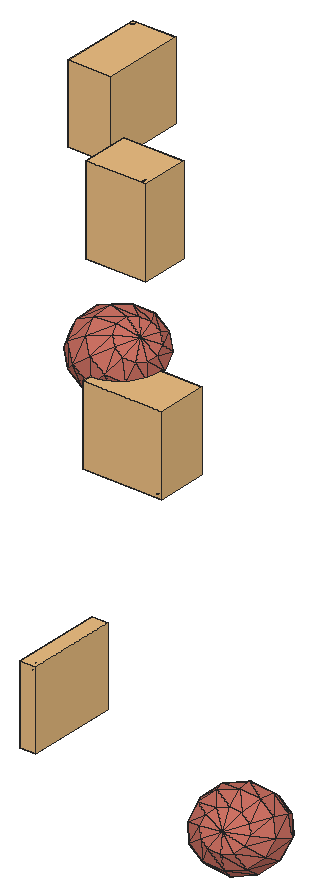
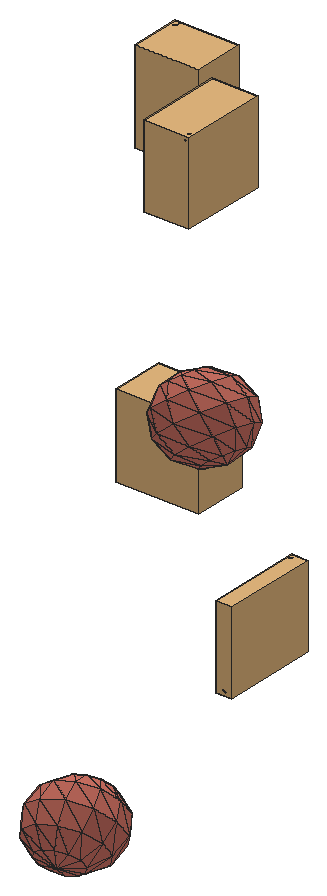
# SketchUp Ruby script. Lengths in inches.
U = 1.inch
M = Sketchup.active_model
def pt(a) = Geom::Point3d.new(a.map { |v| v * U })
def face(e, loops, mat)
  f = e.add_face(loops[0].map { |a| pt(a) })
  loops[1..].each { |l| e.add_face(l.map { |a| pt(a) }).erase! }
  f.material = f.back_material = mat if mat
  f
end
# faces: each face lists its corners as indices into pts; further lists are holes
def faces(e, pts, list, mat = nil) = list.each { |f| face(e, (f[0].is_a?(Array) ? f : [f]).map { |l| l.map { |i| pts[i] } }, mat) }
# xy, xz, yz: faces in a plane at the given z, y or x. An outline is a flat list of corners, or four numbers for a rectangle; further outlines are holes
def ring(l) = l.size == 4 ? [[l[0], l[1]], [l[2], l[1]], [l[2], l[3]], [l[0], l[3]]] : l.each_slice(2).to_a
def flat(e, list, mat, &to3) = list.each { |f| face(e, (f[0].is_a?(Array) ? f : [f]).map { |l| ring(l).map { |u, v| to3.(u, v) } }, mat) }
def xy(e, z, list, mat = nil) = flat(e, list, mat) { |x, y| [x, y, z] }
def xz(e, y, list, mat = nil) = flat(e, list, mat) { |x, z| [x, y, z] }
def yz(e, x, list, mat = nil) = flat(e, list, mat) { |y, z| [x, y, z] }
def lines(e, pts, list) = list.each { |a, b| e.add_line(pt(pts[a]), pt(pts[b])) }
# prism: a flat outline (further loops are holes) pulled along v
def prism(e, loops, v, mat = nil)
  f = face(e, loops, mat); d = Geom::Vector3d.new(v.map { |x| x * U })
  f.pushpull(f.normal.samedirection?(d) ? d.length : -d.length)
end
def box(e, o, s, mat = nil) = prism(e, [[o, [o[0] + s[0], o[1], o[2]], [o[0] + s[0], o[1] + s[1], o[2]], [o[0], o[1] + s[1], o[2]]]], [0, 0, s[2]], mat)
def at(x, y, z, deg = 0) = Geom::Transformation.translation(pt([x, y, z])) * Geom::Transformation.rotation(ORIGIN, Z_AXIS, deg.degrees)
def axes(o, x, y, z) = Geom::Transformation.new([*x, 0, *y, 0, *z, 0, *pt(o).to_a, 1])
def part(name) = M.definitions.add(name)
# library, detail: a bought-in or finely detailed component or shape, given as its bounding box
def library(name, o, s) = part(name).tap { |d| box(d.entities, o, s) }
def detail(e, o, s) = box(e.add_group.entities, o, s)
def put(e, d, t, mat = nil) = e.add_instance(d, t).tap { |i| i.material = mat if mat }
def group(e, t, mat = nil) = e.add_group.tap { |g| g.transformation = t; g.material = mat if mat }.entities
root = M.entities
M.materials.add("green").color = [174, 139, 102]
M.materials.add("vio").color = [206, 114, 100]
c1 = library("3DGeom~88_Defintion",[-500,-434.28,-85.45],[1000,868.56,170.9])
c2 = part("3DGeom~89_Defintion")
p = [[-447.25,-432.03,-61.34],[-483.08,-412.0625,-15.87],[-464.16,-414.34,-85.45],[-447.25,-432.03,-61.34],[-464.16,-414.34,-85.45],[-452.93,-424.73,-76.91],
  [-464.16,-414.34,-85.45],[-483.08,-412.0625,-15.87],[-490.54,-395.51,-74.77],[-464.16,-414.34,-85.45],[-477.93,-403.65,-84.67],[-483.08,-412.0625,-15.87],
  [-500,-394.375,-39.98],[-498.62,-392.12,-58.41],[-456.71,-430.89,-26.55],[-447.25,-432.03,-61.34],[-448.63,-434.28,-42.9],[-456.71,-430.89,-26.55],
  [-483.08,-412.0625,-15.87],[-447.25,-432.03,-61.34],[-483.08,-412.0625,-15.87],[-494.3125,-401.67,-24.41],[478.73,421.99,30.62],[484.28,389.18,-27.12],
  [471.28,398.13,-35.42],[478.73,421.99,30.62],[471.28,398.13,-35.42],[459.28,410.27,-34.875],[478.73,421.99,30.62],[459.28,410.27,-34.875],
  [451.5,422.35,-25.63],[478.73,421.99,30.62],[494.79,385.84,-12.2],[484.28,389.18,-27.12],[-483.08,-412.0625,-15.87],[-456.71,-430.89,-26.55],
  [-469.32,-422.76,-16.65],[478.73,421.99,30.62],[451.5,422.35,-25.63],[450.01,431.14,-10.16],[478.73,421.99,30.62],[500,388.98,5.35],
  [494.79,385.84,-12.2],[478.73,421.99,30.62],[450.01,431.14,-10.16],[455.22,434.28,7.39],[478.73,421.99,30.62],[498.51,397.77,20.82],
  [500,388.98,5.35],[478.73,421.99,30.62],[455.22,434.28,7.39],[465.73,430.9375,22.3125],[478.73,421.99,30.62],[490.73,409.85,30.07]]
faces(c2.entities,p,[[0,1,2],[3,4,5],[6,7,8],[9,8,10],[8,11,12],[8,12,13],[14,15,16],[17,18,19],
  [20,21,12],[22,23,24],[25,26,27],[28,29,30],[31,32,33],[34,35,36],[37,38,39],[40,41,42],
  [43,44,45],[46,47,48],[49,50,51],[52,53,47]],"green")
c3 = library("3DGeom~92_Defintion",[-269.59,-500,-344.14],[539.17,1000,688.28])
c4 = part("3DGeom~93_Defintion")
p = [[-217.33,-469.79,-343.43],[-251.16,-458.84,-336.67],[-234.01,-461.98,-344.14],[-217.33,-469.79,-343.43],[-220.35,-500,-290.57],[-251.16,-458.84,-336.67],
  [-201.93,-490.37,-320.375],[-201.93,-490.37,-320.375],[-217.33,-469.79,-343.43],[-205.59,-480.18,-334.73],[-269.59,-468.47,-306.87],[-251.16,-458.84,-336.67],
  [-269.59,-468.47,-306.87],[-264.18,-461.21,-323.03],[-220.35,-500,-290.57],[-201.93,-490.37,-320.375],[-207.33,-497.625,-304.21],[-254.18,-489.05,-283.82],
  [-269.59,-468.47,-306.87],[-254.18,-489.05,-283.82],[-265.93,-478.66,-292.52],[-220.35,-500,-290.57],[-237.5,-496.86,-283.11],[-254.18,-489.05,-283.82],
  [253.72,487.39,337.56],[230.5,498.77,271.66],[212.66,500,278.24],[253.72,487.39,337.56],[249.06,496.1875,274.79],[230.5,498.77,271.66],
  [253.72,487.39,337.56],[263.36,492.93,286.79],[249.06,496.1875,274.79],[253.72,487.39,337.56],[212.66,500,278.24],[200.33,499.54,292.76],
  [253.72,487.39,337.56],[269.58,489.88,304.45],[263.36,492.93,286.79],[253.72,487.39,337.56],[200.33,499.54,292.76],[196.8,497.51,311.34],
  [253.72,487.39,337.56],[266.06,487.85,323.03],[269.58,489.88,304.45],[253.72,487.39,337.56],[196.8,497.51,311.34],[203.02,494.46,329],
  [253.72,487.39,337.56],[203.02,494.46,329],[217.33,491.2,341.01],[253.72,487.39,337.56],[217.33,491.2,341.01],[235.89,488.61,344.14]]
faces(c4.entities,p,[[0,1,2],[3,4,5],[6,4,3],[7,8,9],[5,4,10],[11,12,13],[14,15,16],[10,4,17],
  [18,19,20],[21,22,23],[24,25,26],[27,28,29],[30,31,32],[33,34,35],[36,37,38],[39,40,41],
  [42,43,44],[45,46,47],[48,49,50],[51,52,53]],"green")
c5 = library("3DGeom~80_Defintion",[-319.18,-499.03,-500],[638.36,998.06,1000])
c6 = part("3DGeom~81_Defintion")
p = [[-260.82,484.9,-487.59],[-282.95,457.07,-500],[-298.58,446.97,-491.37],[-260.82,484.9,-487.59],[-269.125,470.95,-498.62],[-282.95,457.07,-500],
  [-260.82,484.9,-487.59],[-298.58,446.97,-491.37],[-311.84,443.35,-475.05],[-260.82,484.9,-487.59],[-311.84,443.35,-475.05],[-319.18,447.2,-455.39],
  [-260.82,484.9,-487.59],[-318.61,457.48,-437.68],[-260.82,484.9,-487.59],[-318.61,457.48,-437.68],[-310.3125,471.43,-426.66],[-260.82,484.9,-487.59],
  [-310.3125,471.43,-426.66],[-296.49,485.3125,-425.27],[-260.82,484.9,-487.59],[-296.49,485.3125,-425.27],[-280.85,495.42,-433.9],[-260.82,484.9,-487.59],
  [-280.85,495.42,-433.9],[-267.59,499.03,-450.23],[-260.82,484.9,-487.59],[-267.59,499.03,-450.23],[-260.26,495.18,-469.88],[291.93,-495.13,436.625],
  [252.8,-496.44,450.23],[271.18,-499.03,439.58],[291.93,-495.13,436.625],[319.18,-473.5,454.71],[252.8,-496.44,450.23],[319.18,-473.5,454.71],
  [291.93,-495.13,436.625],[309.5,-485.78,442.16],[252.8,-496.44,450.23],[319.18,-473.5,454.71],[240.91,-476.12,481.92],[252.8,-496.44,450.23],
  [240.91,-476.12,481.92],[241.72,-488.05,465.72],[240.91,-476.12,481.92],[319.18,-473.5,454.71],[268.15,-454.48,500],[319.18,-473.5,454.71],
  [307.29,-453.17,486.4],[319.18,-473.5,454.71],[318.36,-461.56,470.9],[307.29,-453.17,486.4],[240.91,-476.12,481.92],[250.59,-463.83,494.46],
  [307.29,-453.17,486.4],[288.91,-450.58,497.05]]
faces(c6.entities,p,[[0,1,2],[3,4,5],[6,7,8],[9,10,11],[12,11,13],[14,15,16],[17,18,19],[20,21,22],
  [23,24,25],[26,27,28],[29,30,31],[32,33,34],[35,36,37],[38,39,40],[41,42,43],[44,45,46],
  [46,47,48],[49,50,51],[52,46,53],[46,54,55]],"green")
c7 = part("3DGeom~211_Defintion")
p = [[79.95,87.67,-500],[-17.63,-123.72,-495.48],[-148.11,-102.41,-480.17],[269.72,-13.2,-440.53],[-146.05,124.59,-473.48],[375.23,159.1,-301.875],
  [156.11,275.58,-370.54],[375.23,159.1,-301.875],[156.11,275.58,-370.54],[-110.49,-301.97,-358.2],[91.93,-181.96,-461.15],[-110.49,-301.97,-358.2],
  [-264.54,-123.72,-419.32],[-110.49,-301.97,-358.2],[-264.54,-123.72,-419.32],[-264.54,-123.72,-419.32],[-347.71,87.67,-368.09],[-104.85,318.21,-339.92],
  [-347.71,87.67,-368.09],[156.11,275.58,-370.54],[-104.85,318.21,-339.92],[151.22,-261.51,-386.375],[-110.49,-301.97,-358.2],[372.42,-150.98,-311.01],
  [372.42,-150.98,-311.01],[493.82,0,-152.32],[372.42,-150.98,-311.01],[269.72,-13.2,-440.53],[269.72,-13.2,-440.53],[375.23,159.1,-301.875],
  [-335.73,-181.96,-329.24],[-264.54,-123.72,-419.32],[-110.49,-301.97,-358.2],[-347.71,87.67,-368.09],[-264.54,-123.72,-419.32],[-335.73,-181.96,-329.24],
  [144.36,-341.07,-291.1875],[-110.49,-301.97,-358.2],[360.52,-288.77,-146.15],[360.52,-288.77,-146.15],[372.42,-150.98,-311.01],[380.21,288.77,-82.33],
  [156.11,275.58,-370.54],[190.4375,389.64,-141.8],[156.11,275.58,-370.54],[-104.85,318.21,-339.92],[380.21,288.77,-82.33],[156.11,275.58,-370.54],
  [190.4375,389.64,-141.8],[-471.01,-13.2,-212.05],[-337.71,275.58,-218.22],[-104.85,318.21,-339.92],[-347.71,87.67,-368.09],[-337.71,275.58,-218.22],
  [-43.26,-420.62,-140.25],[-173.74,-399.3,-124.94],[-110.49,-301.97,-358.2],[73.17,-399.3,-201.1],[-283.3,-341.07,-159.28],[144.36,-341.07,-291.1875],
  [-342.59,-261.51,-234.05],[-342.59,-261.51,-234.05],[-335.73,-181.96,-329.24],[-110.49,-301.97,-358.2],[-35.56,426.5625,-115.28],[-337.71,275.58,-218.22],
  [-342.59,-261.51,-234.05],[480.08,-159.1,38.05],[360.52,-288.77,-146.15],[482.9,150.98,47.19],[380.21,288.77,-82.33],[237.22,-389.64,9.88],
  [144.36,-341.07,-291.1875],[237.22,-389.64,9.88],[144.36,-341.07,-291.1875],[360.52,-288.77,-146.15],[-482.9,-150.98,-47.19],[-283.3,-341.07,-159.28],
  [-480.08,159.1,-38.05],[-237.22,389.64,-9.88],[-337.71,275.58,-218.22],[-237.22,389.64,-9.88],[35.56,-426.5625,115.28],[237.22,-389.64,9.88],
  [-380.21,-288.77,82.33],[-283.3,-341.07,-159.28],[-380.21,-288.77,82.33],[471.01,13.2,212.05],[337.71,-275.58,218.22],[237.22,-389.64,9.88],
  [283.3,341.07,159.28],[380.21,288.77,-82.33],[173.74,399.3,124.94],[-190.4375,-389.64,141.8],[-380.21,-288.77,82.33],[43.26,420.62,140.25],
  [342.59,261.51,234.05],[380.21,288.77,-82.33],[342.59,261.51,234.05],[380.21,288.77,-82.33],[283.3,341.07,159.28],[-493.82,0,152.32],
  [-360.52,288.77,146.15],[-237.22,389.64,-9.88],[-360.52,288.77,146.15],[-73.17,399.3,201.1],[-360.52,288.77,146.15],[104.85,-318.21,339.92],
  [237.22,-389.64,9.88],[104.85,-318.21,339.92],[237.22,-389.64,9.88],[337.71,-275.58,218.22],[347.71,-87.67,368.09],[335.73,181.96,329.24],
  [335.73,181.96,329.24],[342.59,261.51,234.05],[-375.23,-159.1,301.875],[-190.4375,-389.64,141.8],[-375.23,-159.1,301.875],[-156.11,-275.58,370.54],
  [-156.11,-275.58,370.54],[104.85,-318.21,339.92],[110.49,301.97,358.2],[110.49,301.97,358.2],[110.49,301.97,358.2],[-375.23,-159.1,301.875],
  [-190.4375,-389.64,141.8],[-156.11,-275.58,370.54],[-360.52,288.77,146.15],[-372.42,150.98,311.01],[-144.36,341.07,291.1875],[-360.52,288.77,146.15],
  [-372.42,150.98,311.01],[-360.52,288.77,146.15],[-144.36,341.07,291.1875],[-372.42,150.98,311.01],[-375.23,-159.1,301.875],[342.59,261.51,234.05],
  [110.49,301.97,358.2],[-144.36,341.07,291.1875],[110.49,301.97,358.2],[264.54,123.72,419.32],[264.54,123.72,419.32],[335.73,181.96,329.24],
  [146.05,-124.59,473.48],[104.85,-318.21,339.92],[337.71,-275.58,218.22],[337.71,-275.58,218.22],[347.71,-87.67,368.09],[335.73,181.96,329.24],
  [342.59,261.51,234.05],[110.49,301.97,358.2],[-151.22,261.51,386.37],[-269.72,13.2,440.53],[-375.23,-159.1,301.875],[-156.11,-275.58,370.54],
  [-372.42,150.98,311.01],[-375.23,-159.1,301.875],[-269.72,13.2,440.53],[264.54,123.72,419.32],[-79.95,-87.67,500],[17.63,123.72,495.48],
  [148.11,102.41,480.17],[-91.93,181.96,461.15],[347.71,-87.67,368.09],[347.71,-87.67,368.09]]
faces(c7.entities,p,[[0,1,2],[3,1,0],[0,2,4],[5,3,0],[6,0,4],[7,0,8],[2,1,9],[1,10,11],
  [3,10,1],[12,2,13],[4,2,14],[4,15,16],[17,4,18],[19,4,20],[10,21,22],[23,21,10],
  [24,10,3],[25,26,27],[25,28,29],[30,31,32],[33,34,35],[21,36,37],[38,36,21],[39,21,40],
  [41,29,42],[43,44,45],[46,47,48],[33,35,49],[50,33,49],[51,52,53],[54,55,56],[57,54,56],
  [55,58,56],[59,57,56],[58,60,56],[61,62,63],[64,45,65],[43,45,64],[49,35,66],[67,68,26],
  [67,26,25],[69,25,29],[69,29,70],[71,57,72],[73,74,75],[76,66,77],[49,66,76],[50,49,78],
  [79,50,78],[64,80,81],[78,49,76],[82,54,57],[82,57,83],[84,58,55],[76,85,86],[87,67,25],
  [87,25,69],[88,89,68],[88,68,67],[90,91,43],[90,43,92],[92,43,64],[93,54,82],[93,55,54],
  [94,55,93],[95,64,81],[92,64,95],[96,69,97],[98,99,100],[101,76,86],[78,76,101],[102,78,101],
  [103,78,104],[105,81,106],[95,81,105],[107,82,108],[109,110,111],[112,88,67],[112,67,87],[113,87,69],
  [114,69,115],[116,86,117],[101,86,118],[119,93,82],[120,82,121],[92,95,122],[90,92,123],[95,105,124],
  [125,126,127],[128,101,129],[130,131,132],[105,133,134],[135,101,136],[137,90,138],[105,139,140],[141,112,87],
  [142,87,143],[144,145,146],[144,147,148],[149,150,151],[130,132,152],[130,152,151],[153,154,155],[156,157,158],
  [152,132,153],[159,149,151],[160,155,145],[160,145,144],[161,162,151],[162,159,151],[163,161,151],[152,163,151],
  [162,144,164],[162,165,159],[153,155,160],[152,153,163],[163,153,160],[163,160,161],[161,160,144],[161,144,162]],"vio")
c8 = part("3DGeom~214_Defintion")
p = [[-289.85,-175.69,-352.13],[-81.66,-101.43,-479.48],[-0.05,-263.22,-393.3125],[242.66,-186.82,-378.86],[-0.05,-263.22,-393.3125],[148.41,0,-478.35],
  [-356.86,-82.28,-337.79],[-289.85,-175.69,-352.13],[-356.86,-82.28,-337.79],[-197.72,60.36,-454.64],[420.34,-60.36,-262.88],[338.72,101.43,-349.05],
  [420.34,-60.36,-262.88],[14.41,186.82,-449.67],[-425.79,-13.9,-263.21],[-356.86,-82.28,-337.79],[-425.79,-13.9,-263.21],[-317.11,178.79,-325.46],
  [222.67,263.22,-324.21],[-123.46,323.58,-300.5],[-242.73,-269.1,-302.38],[-0.05,-263.22,-393.3125],[25.26,-381.66,-219.23],[-0.05,-263.22,-393.3125],
  [271.875,-323.58,-177.85],[25.26,-381.66,-219.23],[-0.05,-263.22,-393.3125],[271.875,-323.58,-177.85],[-289.85,-175.69,-352.13],[-0.05,-263.22,-393.3125],
  [-242.73,-269.1,-302.38],[242.66,-186.82,-378.86],[445.64,-178.79,-88.8],[271.875,-323.58,-177.85],[242.66,-186.82,-378.86],[420.34,-60.36,-262.88],
  [-289.85,-175.69,-352.13],[-242.73,-269.1,-302.38],[-420.38,-202.87,-130.43],[-356.86,-82.28,-337.79],[338.72,101.43,-349.05],[485.39,82.28,-76.47],
  [338.72,101.43,-349.05],[438.27,175.69,-126.22],[222.67,263.22,-324.21],[338.72,101.43,-349.05],[-425.79,-13.9,-263.21],[-478.1875,11.13,-148.36],
  [-317.11,178.79,-325.46],[-407.86,222.15,-126.54],[-317.11,178.79,-325.46],[-407.86,222.15,-126.54],[-123.46,323.58,-300.5],[-317.11,178.79,-325.46],
  [222.67,263.22,-324.21],[371.26,269.1,-111.88],[103.27,381.66,-195.03],[103.27,381.66,-195.03],[371.26,269.1,-111.88],[222.67,263.22,-324.21],
  [-242.73,-269.1,-302.38],[-228.125,-337.48,-201.88],[-228.125,-337.48,-201.88],[-407.86,222.15,-126.54],[-228.25,373.64,-70.82],[-123.46,323.58,-300.5],
  [103.27,381.66,-195.03],[-123.46,323.58,-300.5],[500,13.9,24.03],[-228.125,-337.48,-201.88],[-12.52,-425.01,-3.88],[228.25,-373.64,70.82],
  [271.875,-323.58,-177.85],[-228.125,-337.48,-201.88],[-249.9375,-362.51,-77.55],[-249.9375,-362.51,-77.55],[103.27,381.66,-195.03],[302.33,337.48,-37.3],
  [371.26,269.1,-111.88],[12.52,425.01,3.88],[103.27,381.66,-195.03],[103.27,381.66,-195.03],[271.875,-323.58,-177.85],[407.86,-222.15,126.54],
  [228.25,-373.64,70.82],[271.875,-323.58,-177.85],[-500,-13.9,-24.03],[-302.33,-337.48,37.3],[-371.26,-269.1,111.88],[-438.27,-175.69,126.22],
  [-485.39,-82.28,76.47],[-445.64,178.79,88.8],[-228.25,373.64,-70.82],[420.38,202.87,130.43],[302.33,337.48,-37.3],[478.1875,-11.13,148.36],
  [-249.9375,-362.51,-77.55],[-103.27,-381.66,195.03],[-249.9375,-362.51,-77.55],[-302.33,-337.48,37.3],[-271.875,323.58,177.85],[-228.25,373.64,-70.82],
  [-271.875,323.58,177.85],[302.33,337.48,-37.3],[249.9375,362.51,77.55],[249.9375,362.51,77.55],[123.46,-323.58,300.5],[123.46,-323.58,300.5],
  [-271.875,323.58,177.85],[-25.26,381.66,219.23],[-302.33,-337.48,37.3],[-222.67,-263.22,324.21],[-302.33,-337.48,37.3],[-222.67,-263.22,324.21],
  [-371.26,-269.1,111.88],[317.11,-178.79,325.46],[123.46,-323.58,300.5],[407.86,-222.15,126.54],[317.11,-178.79,325.46],[-420.34,60.36,262.88],
  [249.9375,362.51,77.55],[228.125,337.48,201.88],[228.125,337.48,201.88],[-338.72,-101.43,349.05],[-222.67,-263.22,324.21],[425.79,13.9,263.21],
  [317.11,-178.79,325.46],[425.79,13.9,263.21],[425.79,13.9,263.21],[356.86,82.28,337.79],[425.79,13.9,263.21],[289.85,175.69,352.13],
  [356.86,82.28,337.79],[242.73,269.1,302.38],[289.85,175.69,352.13],[228.125,337.48,201.88],[242.73,269.1,302.38],[-242.66,186.82,378.85],
  [-242.66,186.82,378.85],[-25.26,381.66,219.23],[-271.875,323.58,177.85],[-103.27,-381.66,195.03],[-14.41,-186.82,449.67],[-222.67,-263.22,324.21],
  [-103.27,-381.66,195.03],[123.46,-323.58,300.5],[0.05,263.22,393.3125],[0.05,263.22,393.3125],[242.73,269.1,302.38],[-242.66,186.82,378.85],
  [0.05,263.22,393.3125],[-25.26,381.66,219.23],[-338.72,-101.43,349.05],[-242.66,186.82,378.85],[-420.34,60.36,262.88],[317.11,-178.79,325.46],
  [425.79,13.9,263.21],[356.86,82.28,337.79],[197.71,-60.36,454.64],[81.66,101.43,479.48],[242.73,269.1,302.38],[289.85,175.69,352.13],
  [242.73,269.1,302.38],[-222.67,-263.22,324.21],[-148.41,0,478.35],[-338.72,-101.43,349.05],[-222.67,-263.22,324.21],[-338.72,-101.43,349.05],
  [-242.66,186.82,378.85],[-242.66,186.82,378.85]]
faces(c8.entities,p,[[0,1,2],[1,3,4],[1,5,3],[6,1,7],[8,9,1],[9,5,1],[5,10,3],[5,11,12],
  [9,13,5],[13,11,5],[14,9,15],[16,17,9],[17,13,9],[13,18,11],[17,19,13],[19,18,13],
  [20,21,22],[23,24,25],[26,3,27],[28,29,30],[31,32,33],[34,35,32],[36,37,38],[39,36,38],
  [40,41,35],[42,43,41],[44,43,45],[46,39,38],[47,48,46],[47,49,50],[51,52,53],[54,55,43],
  [19,56,18],[57,58,59],[60,22,61],[37,62,38],[63,64,65],[64,66,67],[47,46,38],[35,68,32],
  [35,41,68],[69,22,70],[22,71,70],[22,72,71],[73,70,74],[62,75,38],[76,77,78],[79,77,80],
  [64,79,81],[82,83,84],[85,32,83],[86,47,38],[86,49,47],[75,87,38],[87,88,38],[88,89,38],
  [90,86,38],[89,90,38],[86,91,49],[91,92,49],[41,43,93],[43,55,93],[55,94,93],[32,95,83],
  [32,68,95],[96,70,97],[98,97,99],[68,41,93],[91,100,101],[102,79,64],[103,104,93],[79,105,77],
  [90,91,86],[70,106,97],[70,71,107],[108,109,79],[109,105,79],[95,68,93],[110,97,111],[112,113,114],
  [71,115,116],[71,117,118],[89,119,90],[90,119,91],[120,121,93],[109,122,105],[119,100,91],[88,123,89],
  [88,124,123],[89,123,119],[83,125,126],[83,95,127],[128,95,93],[129,130,93],[131,132,93],[133,134,93],
  [135,136,93],[119,137,100],[138,139,140],[141,142,143],[144,145,142],[146,122,109],[147,148,122],[149,150,151],
  [152,153,154],[155,156,157],[145,158,142],[145,155,158],[159,160,150],[159,161,162],[163,164,165],[166,142,164],
  [155,157,158],[158,157,161],[167,164,168],[158,161,159],[164,150,169],[164,159,150],[142,159,164],[142,158,159]],"vio")
c9 = library("3DGeom~61_Defintion",[-500,-478.45,-265.375],[1000,956.89,530.75])
c10 = part("3DGeom~62_Defintion")
p = [[-465.47,464.9,-258.6875],[-477.89,451.53,-263.24],[-489.74,438.22,-257.15],[-465.47,464.9,-258.6875],[-497.83,428.53,-242.0625],[-500,425.07,-222.01],
  [-465.47,464.9,-258.6875],[-500,425.07,-222.01],[-495.67,428.76,-202.375],[-465.47,464.9,-258.6875],[-489.74,438.22,-257.15],[-497.83,428.53,-242.0625],
  [-465.47,464.9,-258.6875],[-495.67,428.76,-202.375],[-485.99,438.61,-188.41],[-465.47,464.9,-258.6875],[-485.99,438.61,-188.41],[-473.5625,451.98,-183.86],
  [-465.47,464.9,-258.6875],[-473.5625,451.98,-183.86],[-461.72,465.3,-189.95],[-465.47,464.9,-258.6875],[-453.625,474.98,-205.04],[-451.46,478.44,-225.09],
  [-465.47,464.9,-258.6875],[-451.46,478.44,-225.09],[-455.79,474.75,-244.72],[-465.47,464.9,-258.6875],[-461.72,465.3,-189.95],[-453.625,474.98,-205.04],
  [492.22,-453.97,197.65],[460.87,-474.71,197.28],[477.9,-465.75,192.59],[460.87,-474.71,197.28],[436.46,-475.96,228.62],[445.7,-478.45,210.47],
  [460.87,-474.71,197.28],[492.22,-453.97,197.65],[436.46,-475.96,228.62],[436.46,-475.96,228.62],[492.22,-453.97,197.65],[443.4,-456.48,260.3125],
  [443.4,-456.48,260.3125],[492.22,-453.97,197.65],[474.74,-435.74,260.68],[474.74,-435.74,260.68],[492.22,-453.97,197.65],[499.15,-434.48,229.35],
  [492.22,-453.97,197.65],[500,-442.52,211.1],[499.15,-434.48,229.35],[436.46,-475.96,228.62],[443.4,-456.48,260.3125],[435.62,-467.92,246.86],
  [474.74,-435.74,260.68],[499.15,-434.48,229.35],[489.91,-432,247.49],[443.4,-456.48,260.3125],[474.74,-435.74,260.68],[457.72,-444.7,265.375]]
faces(c10.entities,p,[[0,1,2],[3,4,5],[6,7,8],[9,10,11],[12,13,14],[15,16,17],[18,19,20],[21,22,23],
  [24,25,26],[27,28,29],[30,31,32],[33,34,35],[36,37,38],[39,40,41],[42,43,44],[45,46,47],
  [48,49,50],[51,52,53],[54,55,56],[57,58,59]],"green")
g1 = group(root,at(15.3125,38.42,26.21))
put(g1,c1,axes([-1.27,-0.22,10.39],[0,0.00041,0],[0,0,-0.00041],[-0.00041,0,0]),"green")
put(g1,c2,axes([-1.27,-0.22,10.39],[0,0.00041,0],[0,0,-0.00041],[-0.00041,0,0]),"green")
g2 = group(root,at(15.3125,38.42,26.21))
put(g2,c3,axes([-1.01,-0.14,12.39],[0,0.0004,0],[0,0,-0.0004],[-0.0004,0,0]),"green")
put(g2,c4,axes([-1.01,-0.14,12.39],[0,0.0004,0],[0,0,-0.0004],[-0.0004,0,0]),"green")
g3 = group(root,at(15.3125,38.42,26.21))
put(g3,c5,axes([-1.23,0.18,11.28],[0,0.00036,0],[0,0,-0.00036],[-0.00036,0,0]),"green")
put(g3,c6,axes([-1.23,0.18,11.28],[0,0.00036,0],[0,0,-0.00036],[-0.00036,0,0]),"green")
g4 = group(root,at(15.3125,38.42,26.21))
put(g4,c7,axes([-1.43,0.29,11.48],[0,0.00038,0],[0,0,-0.00038],[-0.00038,0,0]),"vio")
g5 = group(root,at(15.3125,38.42,26.21))
put(g5,c8,axes([-0.88,0.3,9.71],[0,0.00039,0],[0,0,-0.00039],[-0.00039,0,0]),"vio")
g6 = group(root,at(15.3125,38.42,26.21))
put(g6,c9,axes([-1.4375,0.32,12.52],[0,0.00037,0],[0,0,-0.00037],[-0.00037,0,0]),"green")
put(g6,c10,axes([-1.4375,0.32,12.52],[0,0.00037,0],[0,0,-0.00037],[-0.00037,0,0]),"green")
